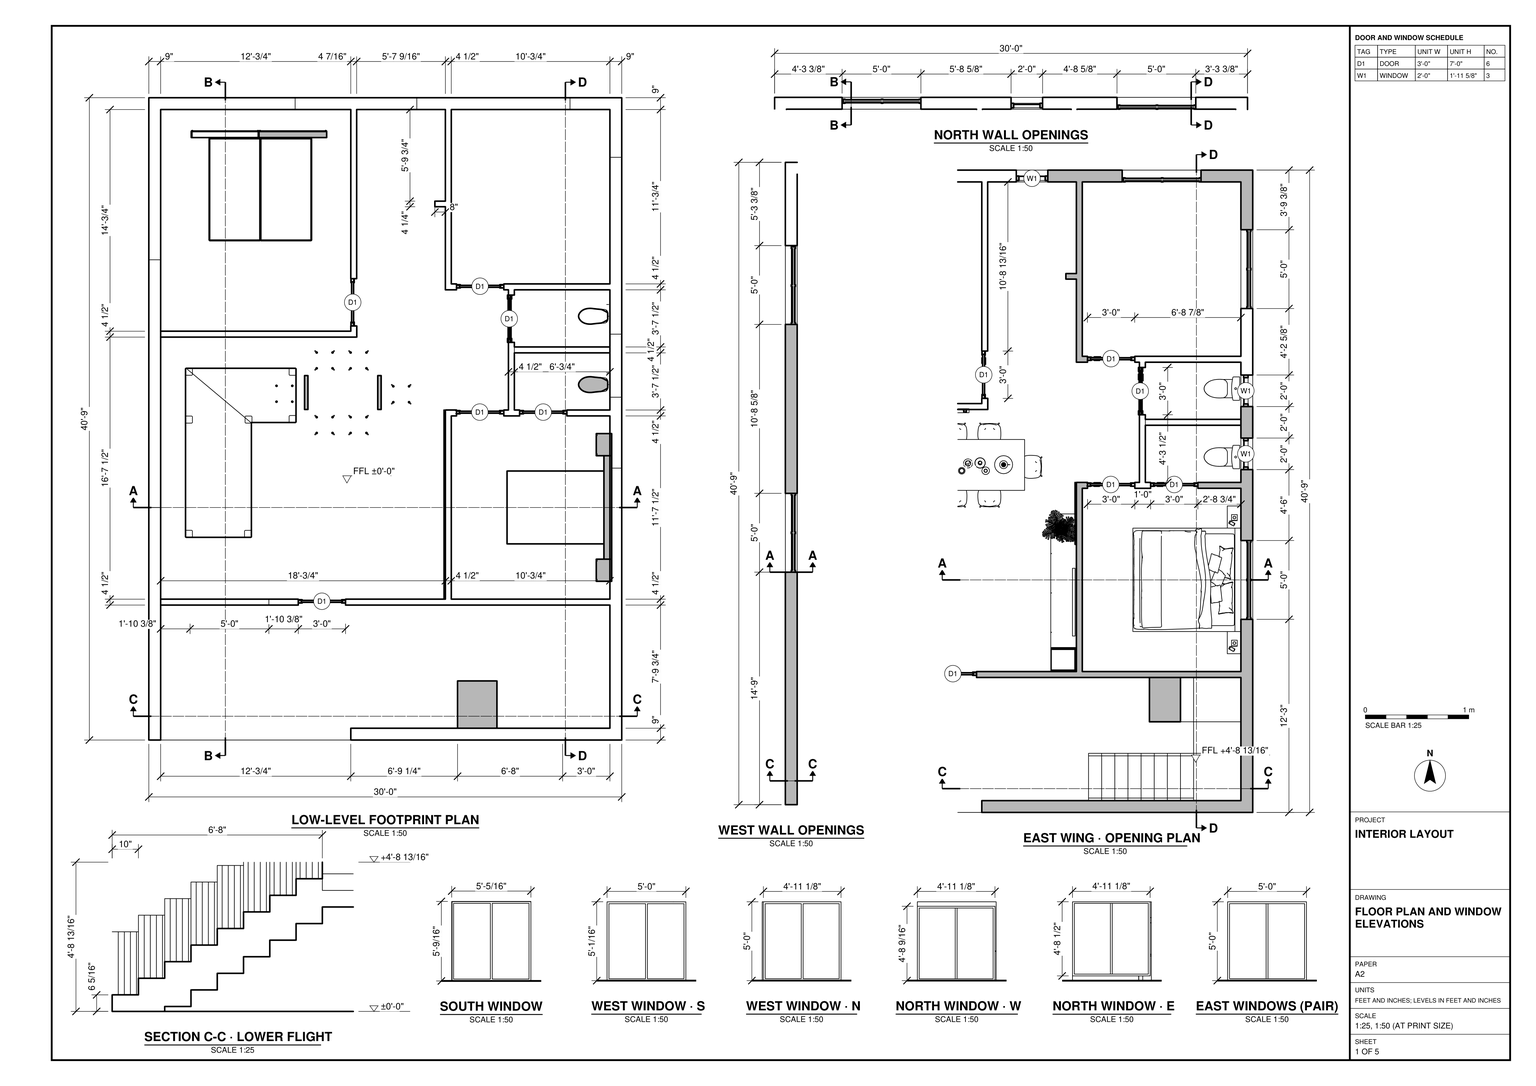
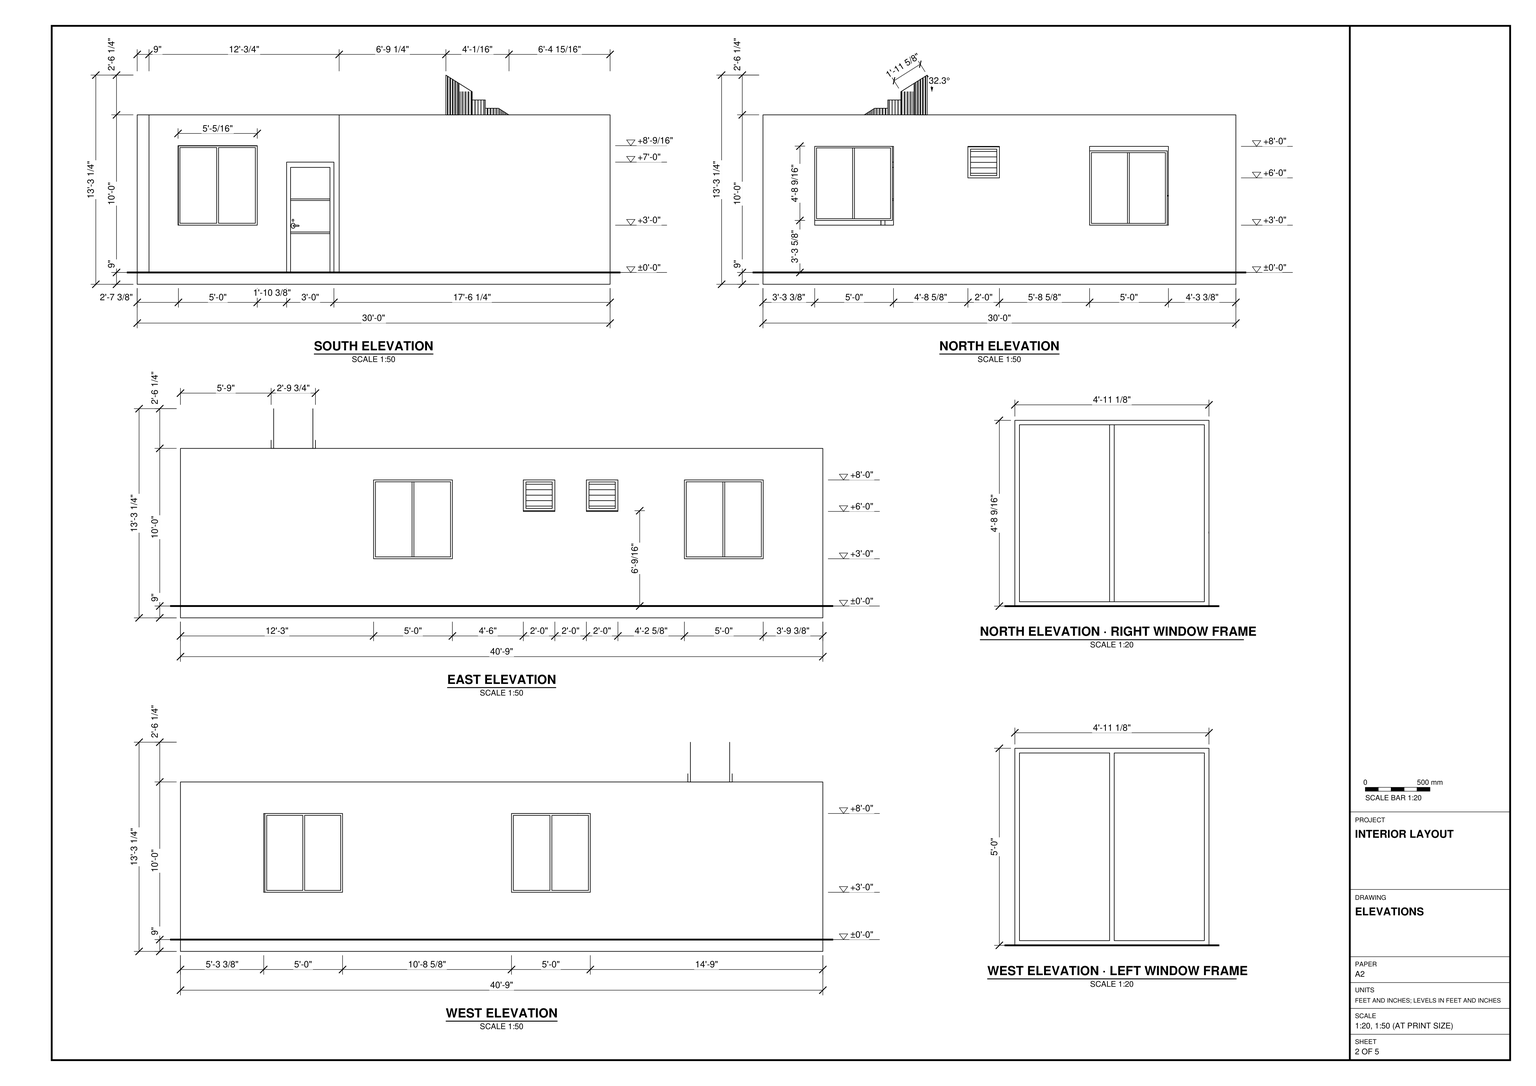
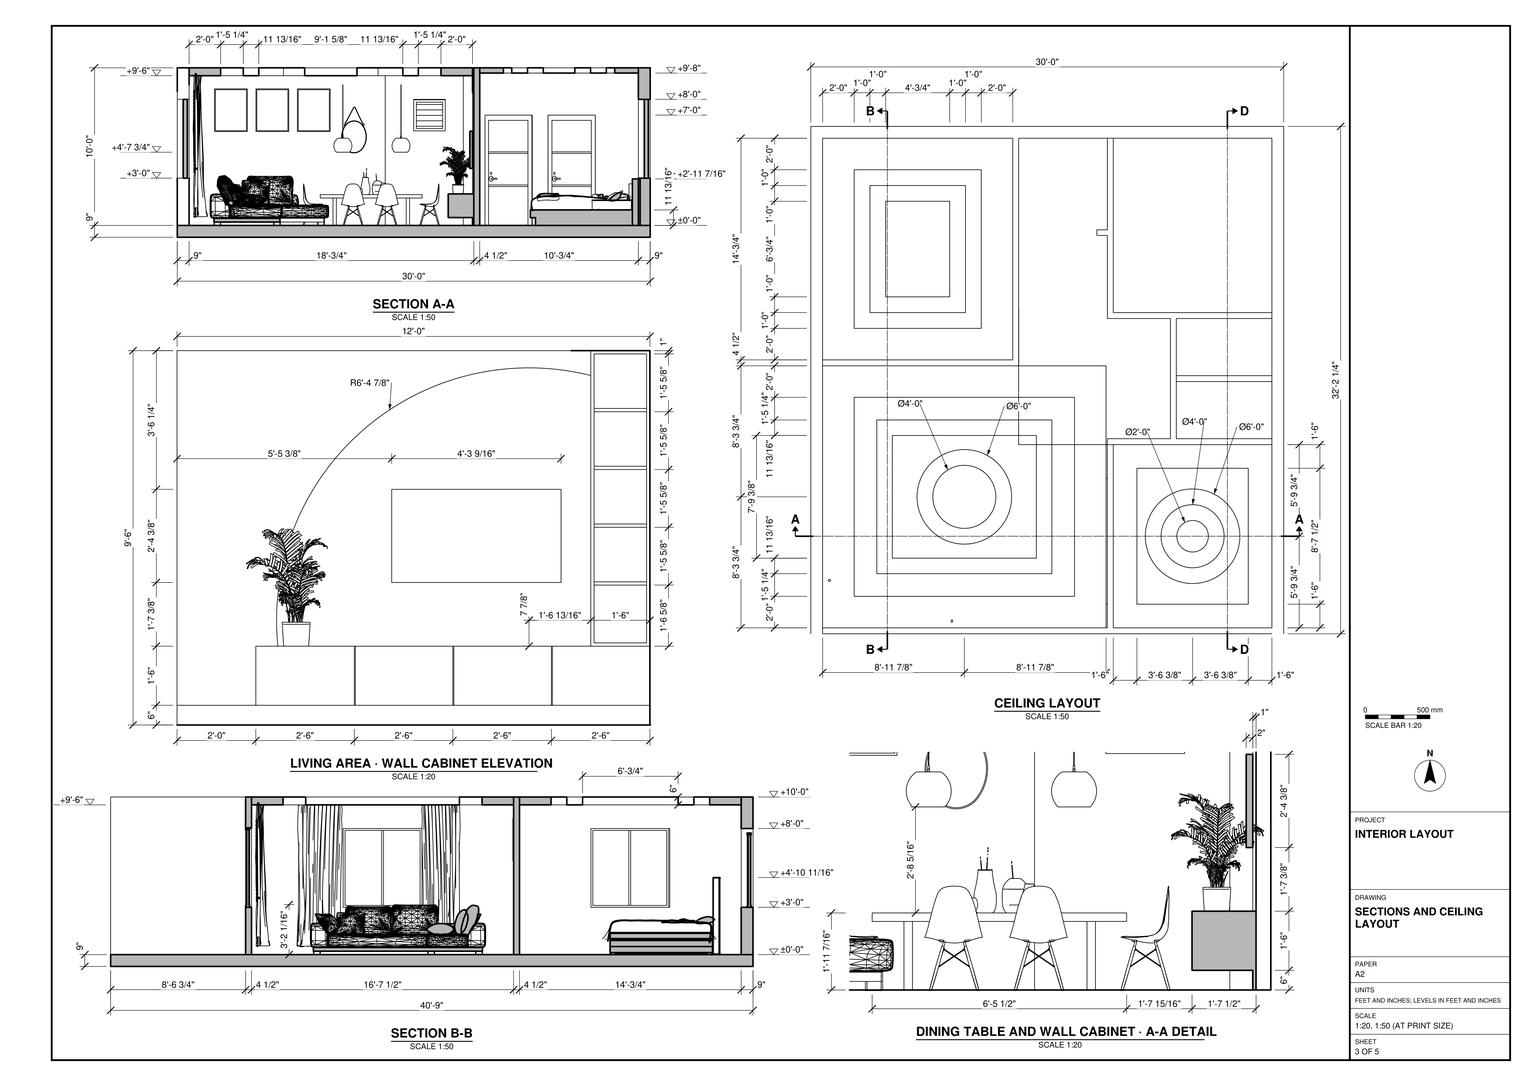
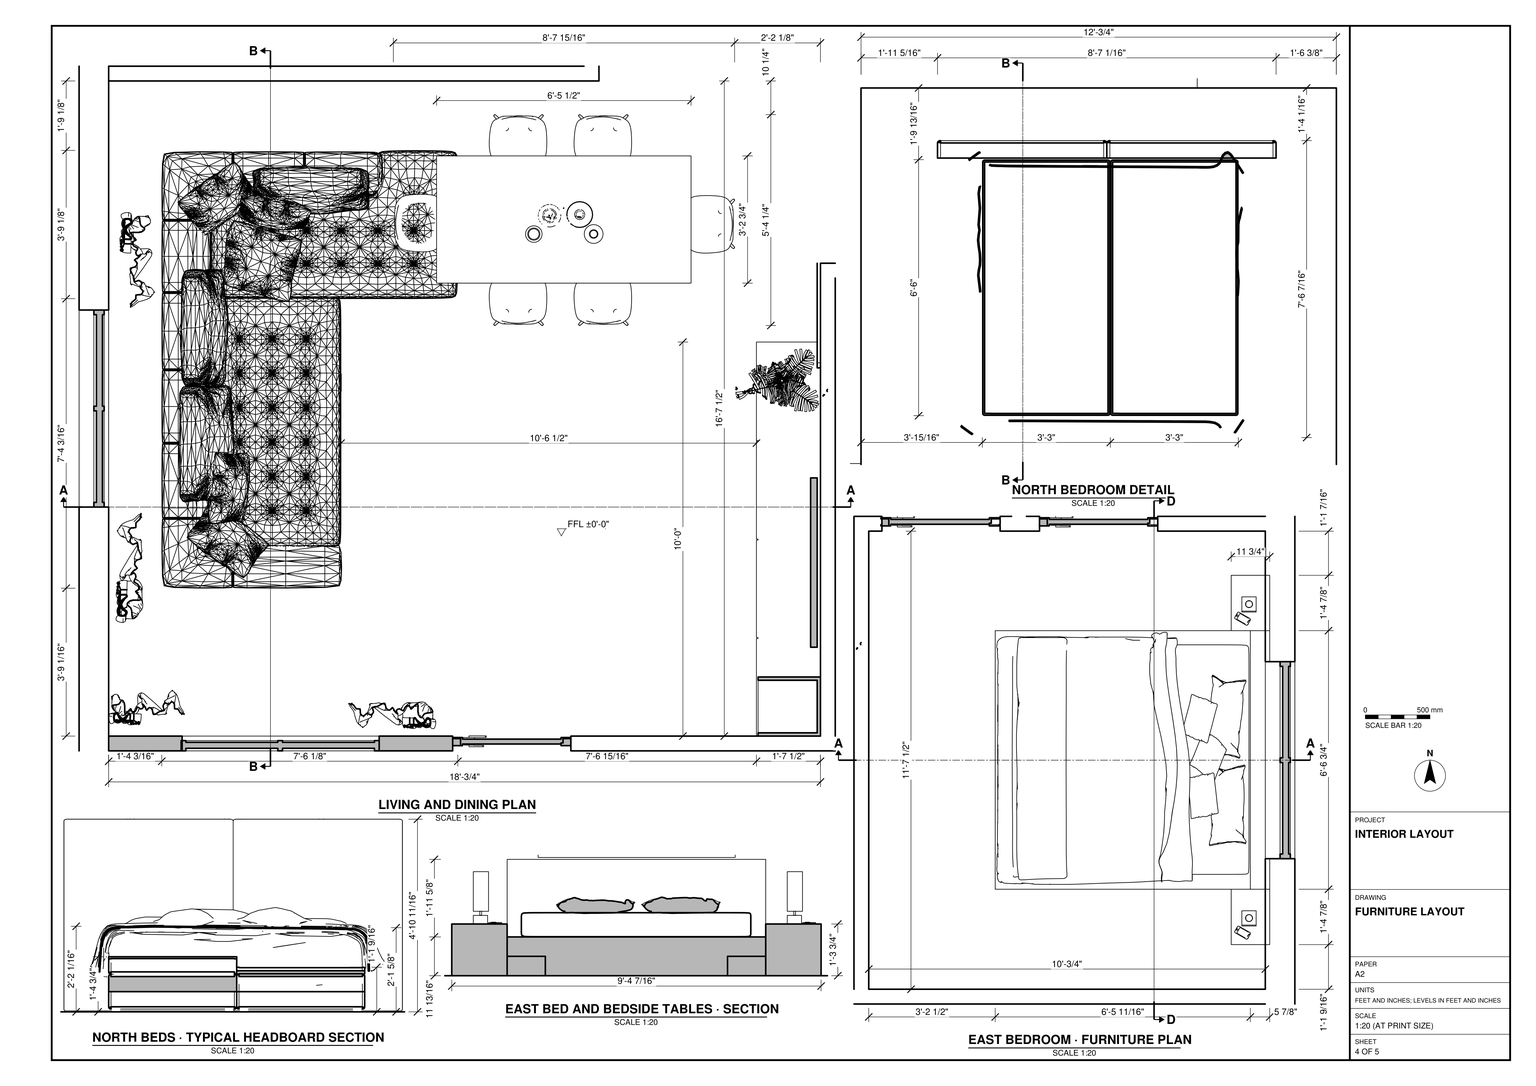
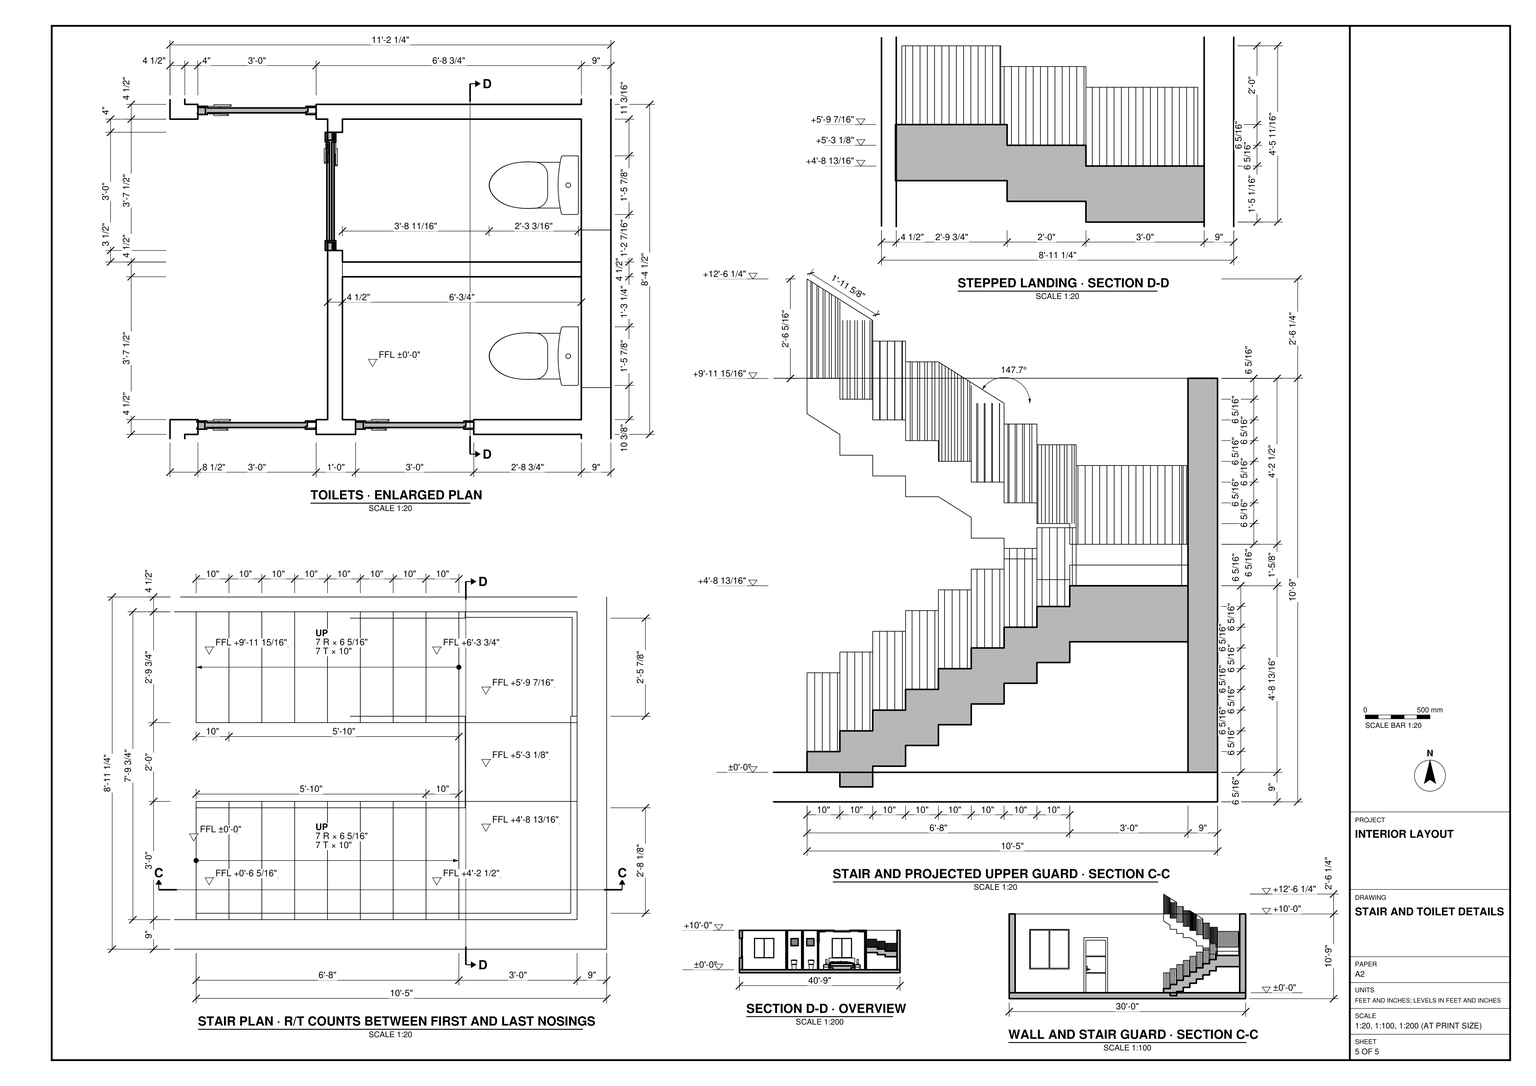
Build the single-storey interior in SketchUp from task_files/diagram_01.pdf. Work in feet and inches. Set the finished floor at ±0'-0" and make the overall model 30'-0" east to west, 40'-9" north to south and 10'-9" high.

Lay out the floor slab, perimeter walls and partitions using the thicknesses on the plan and sections. Keep the living and dining area open on the west side. Place the northwest bed against the north wall and the southeast bed against the east wall. Follow the east-wing plan for the northeast room, the two small toilet rooms and their doorways. Fit the doors and window units, using the elevations to distinguish the large two-panel windows from the smaller high-level openings. Model the lower stair flight, landing and railing in the southern entrance area.

Use the furniture footprints to place the L-shaped sofa, dining table and chairs. Build the living-area wall cabinet with its low cupboards, curved panel edge and tall shelving at one end. Model the flat roof and the changes in ceiling profile, including the nested rectangular and circular features shown in the ceiling plan. Decor and loose items may be any suitable library components.

Keep walls, slabs and roof in separate groups or components, do the same for each furniture or joinery piece, and use components for repeated parts. Save one SketchUp model as output_files/furnished_residential_interior_and_its_entrance_stair.skp.

# SketchUp Ruby script. Lengths in inches.
U = 1.inch
M = Sketchup.active_model
def pt(a) = Geom::Point3d.new(a.map { |v| v * U })
def face(e, loops, mat)
  f = e.add_face(loops[0].map { |a| pt(a) })
  loops[1..].each { |l| e.add_face(l.map { |a| pt(a) }).erase! }
  f.material = f.back_material = mat if mat
  f
end
# faces: each face lists its corners as indices into pts; further lists are holes
def faces(e, pts, list, mat = nil) = list.each { |f| face(e, (f[0].is_a?(Array) ? f : [f]).map { |l| l.map { |i| pts[i] } }, mat) }
# xy, xz, yz: faces in a plane at the given z, y or x. An outline is a flat list of corners, or four numbers for a rectangle; further outlines are holes
def ring(l) = l.size == 4 ? [[l[0], l[1]], [l[2], l[1]], [l[2], l[3]], [l[0], l[3]]] : l.each_slice(2).to_a
def flat(e, list, mat, &to3) = list.each { |f| face(e, (f[0].is_a?(Array) ? f : [f]).map { |l| ring(l).map { |u, v| to3.(u, v) } }, mat) }
def xy(e, z, list, mat = nil) = flat(e, list, mat) { |x, y| [x, y, z] }
def xz(e, y, list, mat = nil) = flat(e, list, mat) { |x, z| [x, y, z] }
def yz(e, x, list, mat = nil) = flat(e, list, mat) { |y, z| [x, y, z] }
def lines(e, pts, list) = list.each { |a, b| e.add_line(pt(pts[a]), pt(pts[b])) }
# prism: a flat outline (further loops are holes) pulled along v
def prism(e, loops, v, mat = nil)
  f = face(e, loops, mat); d = Geom::Vector3d.new(v.map { |x| x * U })
  f.pushpull(f.normal.samedirection?(d) ? d.length : -d.length)
end
def box(e, o, s, mat = nil) = prism(e, [[o, [o[0] + s[0], o[1], o[2]], [o[0] + s[0], o[1] + s[1], o[2]], [o[0], o[1] + s[1], o[2]]]], [0, 0, s[2]], mat)
def at(x, y, z, deg = 0) = Geom::Transformation.translation(pt([x, y, z])) * Geom::Transformation.rotation(ORIGIN, Z_AXIS, deg.degrees)
def axes(o, x, y, z) = Geom::Transformation.new([*x, 0, *y, 0, *z, 0, *pt(o).to_a, 1])
def part(name) = M.definitions.add(name)
# library, detail: a bought-in or finely detailed component or shape, given as its bounding box
def library(name, o, s) = part(name).tap { |d| box(d.entities, o, s) }
def detail(e, o, s) = box(e.add_group.entities, o, s)
def put(e, d, t, mat = nil) = e.add_instance(d, t).tap { |i| i.material = mat if mat }
def group(e, t, mat = nil) = e.add_group.tap { |g| g.transformation = t; g.material = mat if mat }.entities
root = M.entities
M.materials.add("F10").color = [176, 183, 172]
M.materials.add("F11").color = [173, 179, 169]
M.materials.add("F20").color = [169, 167, 158]
M.materials.add("Querkus Oak Naturel Adagio _ Architonic1").color = [173, 130, 81]
M.materials.add("[0010_Snow]").color = [255, 250, 250]
M.materials.add("[0035_Tan]").color = [210, 180, 140]
M.materials.add("[0057_DarkKhaki]").color = [189, 183, 107]
M.materials.add("[0072_DarkSeaGreen]").color = [143, 188, 143]
M.materials.add("[0110_LightSlateGray]").color = [119, 136, 153]
M.materials.add("[Carrera Marble]").color = [207, 207, 207]
M.materials.add("[Color_008]").color = [30, 30, 30]
M.materials.add("[Color_009]").color = [0, 0, 0]
M.materials.add("[Stone Vein Gray]").color = [166, 165, 165]
M.materials.add("[Translucent Glass Gray]").color = [128, 128, 128]
M.materials.add("[Translucent Glass Tinted]1").color = [7, 201, 240]
M.materials.add("[Translucent_Glass_Gray]").color = [128, 128, 128]
M.materials.add("[Wood Cherry Original]").color = [152, 86, 42]
M.materials.add("[Wood Floor Parquet]").color = [145, 89, 39]
c1 = library("main+door",[0,-0.79,0],[47.24,7.88,82.68])
c2 = library("Modern+dining",[-0.9,-1.38,-0.1],[126.72,78.33,130.86])
c3 = library("Senza",[-40.91,-66.2,-0.5],[133.3,90.15,38.26])
c4 = library("Bed",[-100.55,9.74,0],[90.43,103.1,58.68])
c5 = library("Platform bed",[0,0,0],[83.59,112.46,35.43])
c6 = library("CS300DRT",[0,0,0],[27.18,17.85,30.31])
c7 = library("SKT_Nearly Natural 5' Kentia Palm Silk Tree",[-23.18,-17.61,0],[47.48,43.95,59.125])
c8 = library("Curtains and rod",[2.63,-1.46,0.02],[153.32,14.02,114.15])
c9 = part("Group\#37")
prism(c9.entities,[[[0,0.6,0],[0,0.6,24.5],[19,0.6,24.5],[19,0.6,0]],[[0.5,0.6,0.5],[18.5,0.6,0.5],[18.5,0.6,24],[0.5,0.6,24]]],[0,-0.6,0])
c10 = part("F9")
g1 = group(c10.entities,at(48,0,0))
xy(g1,0.5,[[0.5,0.3,18.5,0.6]])
xy(g1,24,[[0.5,0.3,18.5,0.6]])
xz(g1,0.3,[[0.5,0.5,18.5,24]],"F11")
xz(g1,0.6,[[0.5,0.5,18.5,24]],"[0010_Snow]")
yz(g1,0.5,[[0.3,0.5,0.6,24]])
yz(g1,18.5,[[0.3,0.5,0.6,24]])
put(g1,c9,axes([19,0,0],[-1,0,0],[0,1,0],[0,0,1]),"Querkus Oak Naturel Adagio _ Architonic1")
g2 = group(c10.entities,at(24,0,0))
xy(g2,0.5,[[0.5,0.3,18.5,0.6]])
xy(g2,24,[[0.5,0.3,18.5,0.6]])
xz(g2,0.3,[[0.5,0.5,18.5,24]],"F10")
xz(g2,0.6,[[0.5,0.5,18.5,24]],"[0010_Snow]")
yz(g2,0.5,[[0.3,0.5,0.6,24]])
yz(g2,18.5,[[0.3,0.5,0.6,24]])
put(g2,c9,axes([19,0,0],[-1,0,0],[0,1,0],[0,0,1]),"Querkus Oak Naturel Adagio _ Architonic1")
g3 = group(c10.entities,at(0,0,0))
xy(g3,0.5,[[0.5,0.3,18.5,0.6]])
xy(g3,24,[[0.5,0.3,18.5,0.6]])
xz(g3,0.3,[[0.5,0.5,18.5,24]],"F20")
xz(g3,0.6,[[0.5,0.5,18.5,24]],"[0010_Snow]")
yz(g3,0.5,[[0.3,0.5,0.6,24]])
yz(g3,18.5,[[0.3,0.5,0.6,24]])
put(g3,c9,axes([19,0,0],[-1,0,0],[0,1,0],[0,0,1]),"Querkus Oak Naturel Adagio _ Architonic1")
c11 = library("Round wall hanging",[0,0,0],[26.88,1.18,49.49])
c12 = library("Group\#5",[0,0,0],[116.44,93.99,154.6875])
c13 = part("ventilator")
g4 = group(c13.entities,at(0,0,0))
xy(g4,0,[[0,0,24,1],[0,1,24,6.83]],"[Wood Floor Parquet]")
xy(g4,1.75,[[2,0,22,6.83]],"[Wood Floor Parquet]")
xy(g4,21.87,[[2,0,22,6.83]],"[Wood Cherry Original]")
xy(g4,23.62,[[0,0,24,1],[0,1,24,6.83]],"[Wood Floor Parquet]")
xz(g4,0,[[[0,0,24,23.62],[2,1.75,22,21.87]]],"[Wood Floor Parquet]")
xz(g4,6.83,[[[0,0,24,23.62],[2,1.75,22,21.87]]],"[Wood Cherry Original]")
yz(g4,0,[[0,0,1,23.62],[1,0,6.83,23.62]],"[Wood Floor Parquet]")
yz(g4,2,[[0,1.75,6.83,1.75,6.83,7.66,0,3.5],[0,3.5,6.83,7.66,6.83,11.8125,0,7.66],[0,7.66,6.83,11.8125,6.83,15.97,0,11.8125],[0,11.8125,6.83,15.97,6.83,20.12,0,15.97],[0,15.97,6.83,20.12,6.83,21.87,0,21.87]],"[Wood Floor Parquet]")
yz(g4,22,[[0,1.75,0,3.5,6.83,7.66,6.83,1.75],[0,3.5,0,7.66,6.83,11.8125,6.83,7.66],[0,7.66,0,11.8125,6.83,15.97,6.83,11.8125],[0,11.8125,0,15.97,6.83,20.12,6.83,15.97],[0,15.97,0,21.87,6.83,21.87,6.83,20.12]],"[Wood Floor Parquet]")
yz(g4,24,[[0,0,1,23.62],[1,0,6.83,23.62]],"[Wood Floor Parquet]")
p = [[2,0,3.5],[2,6.83,7.66],[22,6.83,7.66],[22,0,3.5],[2,6.83,11.8125],[2,0,7.66],
  [22,0,7.66],[22,6.83,11.8125],[2,0,11.8125],[2,6.83,15.97],[22,6.83,15.97],[22,0,11.8125],
  [2,6.83,20.12],[2,0,15.97],[22,0,15.97],[22,6.83,20.12]]
faces(g4,p,[[0,1,2,3],[4,5,6,7],[8,9,10,11]],"[Translucent Glass Tinted]1")
faces(g4,p,[[12,13,14,15]],"[Translucent Glass Gray]")
c14 = part("Group\#2")
xy(c14.entities,0,[[0,0,82.68,1.18]],"[Color_009]")
xy(c14.entities,1.97,[[1.97,0.98,40.35,1.18],[42.32,0.98,80.71,1.18]])
xy(c14.entities,1.97,[[1.97,0,40.35,0.3],[42.32,0,80.71,0.3]],"[Color_009]")
xy(c14.entities,80.71,[[1.97,0,40.35,0.3],[42.32,0,80.71,0.3],[1.97,0.3,40.35,0.98],[42.32,0.3,80.71,0.98],[1.97,0.98,40.35,1.18],
  [42.32,0.98,80.71,1.18]])
xy(c14.entities,82.68,[[0,0,82.68,1.18]],"[Color_008]")
xz(c14.entities,0,[[[0,0,82.68,82.68],[1.97,1.97,40.35,80.71],[42.32,1.97,80.71,80.71]]],"[Color_009]")
xz(c14.entities,0.3,[[1.97,1.97,40.35,80.71],[42.32,1.97,80.71,80.71]],"[Translucent_Glass_Gray]")
xz(c14.entities,0.98,[[1.97,1.97,40.35,80.71],[42.32,1.97,80.71,80.71]],"[Translucent_Glass_Gray]")
xz(c14.entities,1.18,[[[0,0,82.68,82.68],[1.97,1.97,80.71,80.71]],[40.35,1.97,42.32,80.71]],"[Color_009]")
yz(c14.entities,0,[[0,0,1.18,82.68]],"[Color_009]")
yz(c14.entities,1.97,[[0.98,1.97,1.18,80.71]])
yz(c14.entities,1.97,[[0,1.97,0.3,80.71]],"[Color_009]")
yz(c14.entities,40.35,[[0,1.97,0.3,80.71],[0.98,1.97,1.18,80.71]],"[Color_009]")
yz(c14.entities,42.32,[[0,1.97,0.3,80.71],[0.98,1.97,1.18,80.71]])
yz(c14.entities,80.71,[[0,1.97,0.3,80.71],[0.98,1.97,1.18,80.71]],"[Color_009]")
yz(c14.entities,82.68,[[0,0,1.18,82.68]],"[Color_009]")
c15 = library("Group\#28",[0,0,0],[19.5,144,120])
c16 = library("Group\#36",[0,0,-6],[215.75,199.5,6])
c17 = library("Group\#42",[0,0,-4],[120.75,139.5,4])
xy(root,120,[[158.21,246.75,351,246.75,351,347.25,230.25,347.25,230.25,480,158.21,480],[230.25,347.25,351,480]])
# 2 loose lines left out
put(root,c1,axes([282.21,248.34,0],[0.762,0,0],[0,0.42,0],[0,0,1.016]))
put(root,c1,axes([233.96,248.34,0],[0.762,0,0],[0,0.42,0],[0,0,1.016]))
put(root,c1,axes([273.75,338.75,0],[0,-0.762,0],[0.42,0,0],[0,0,1.016]))
put(root,c2,axes([96.43,233.41,-0.1],[0.82,0,0],[0,0.82,0],[0,0,0.82]))
put(root,c3,at(49.13,193.21,0.31,90))
put(root,c4,at(22.55,363.42,0,-90))
put(root,c5,at(268.76,120.84,0))
put(root,c6,at(350.09,331.57,0,180))
put(root,c6,at(350.09,279.51,0,180))
put(root,c7,axes([213.79,214.89,23.75],[0.65,0,0],[0,0.65,0],[0,0,0.65]))
put(root,c8,axes([7.29,108.71,5.83],[0.65,0,0],[0,1,0],[0,0,1]))
put(root,c8,axes([10.46,268.91,5.83],[0,-0.8151,0],[1,0,0],[0,0,1]))
put(root,c10,axes([28.35,306.15,71.47],[1.3144,0,0],[0,1.24,0],[0,0,1.3268]))
put(root,c11,axes([124.94,304.29,55.15],[0.71,0,0],[0,2.5702,0],[0,0,0.71]))
put(root,c12,at(235,9,-4.4375))
g5 = group(root,at(0,0,-9))
xy(g5,0,[[0,0,360,489]])
xy(g5,9,[[0,0,360,489]],"[Stone Vein Gray]")
xz(g5,0,[[0,0,360,9]])
xz(g5,489,[[0,0,360,9]])
yz(g5,0,[[0,0,489,9]])
yz(g5,360,[[0,0,489,9]])
g6 = group(root,at(0,0,0))
xy(g6,0,[[0,0,9,177],[153.75,0,153.75,9,351,9,351,102.75,149.75,102.75,149.75,107.25,225.75,107.25,225.75,251.25,234.25,251.25,234.25,246.75,230.25,246.75,230.25,107.25,351,107.25,351,207,360,207,360,0],[9,102.75,91.375,107.25],[91.375,102.75,113.75,107.25],[0,177,9,365.625],
  [351,207,351,246.75,318.25,246.75,318.25,251.25,351,251.25,351,261,360,261,360,207],[270.25,246.75,270.25,251.25,273.75,251.25,273.75,302.75,278.25,302.75,278.25,251.25,282.25,251.25,282.25,246.75],[351,261,360,309],[9,306.75,9,311.25,153.75,311.25,153.75,315.25,158.3,315.25,158.3,306.75],[351,309,351,342.75,278.25,342.75,278.25,338.75,273.75,338.75,273.75,342.75,270.25,342.75,270.25,347.25,351,347.25,351,443.625,360,443.625,360,309],
  [225.75,342.75,225.75,406.01,217.75,406.01,217.75,410.25,225.75,410.25,225.75,480,204,480,204,489,320.625,489,320.625,480,230.25,480,230.25,347.25,234.23,347.25,234.23,342.75],[153.75,351.25,153.75,480,111.375,480,111.375,489,204,489,204,480,158.21,480,158.21,351.25],[0,365.625,0,489,111.375,489,111.375,480,9,480,9,365.625],[351,443.625,351,480,320.625,480,320.625,489,360,489,360,443.625]])
xy(g6,36,[[31.375,102.75,91.375,107.25],[351,147,360,207],[0,177,9,237],[0,365.625,9,425.625],[351,383.625,360,443.625],
  [51.375,480,111.375,489],[260.625,480,320.625,489]])
xy(g6,72,[[351,261,360,285],[351,309,360,333],[180,480,204,489]])
xy(g6,84,[[113.75,102.75,149.75,107.25],[234.25,246.75,270.25,251.25],[282.25,246.75,318.25,251.25],[273.75,302.75,278.25,338.75],[153.75,315.25,158.21,351.25],
  [158.21,315.25,158.3,351.25],[234.23,342.75,270.25,347.25]])
xy(g6,96,[[351,147,360,207],[0,177,9,237],[351,261,360,285],[351,309,360,333],[0,365.625,9,425.625],
  [351,383.625,360,443.625],[51.375,480,111.375,489],[180,480,204,489],[260.625,480,320.625,489]])
xy(g6,96.36,[[31.375,102.75,91.375,107.25]])
xy(g6,120,[[[0,0,9,0,9,480,153.75,480,153.75,311.25,9,311.25,9,306.75,158.3,306.75,158.3,351.25,158.21,351.25,158.21,480,225.75,480,225.75,410.25,217.75,410.25,217.75,406.01,225.75,406.01,225.75,342.75,273.75,342.75,273.75,251.25,225.75,251.25,225.75,107.25,9,107.25,9,102.75,351,102.75,351,9,153.75,9,153.75,0,360,0,360,489,0,489],[230.25,107.25,351,246.75],[230.25,347.25,351,480],[278.25,251.25,351,342.75]],[278.25,294.75,351,299.25]])
xz(g6,0,[[0,0,9,120],[153.75,0,360,120]])
xz(g6,9,[[153.75,0,351,120]])
xz(g6,102.75,[[[9,0,113.75,0,113.75,84,149.75,84,149.75,0,351,0,351,120,9,120],[31.375,36,91.375,96.36]]])
xz(g6,107.25,[[91.375,0,91.375,120,225.75,120,225.75,0,149.75,0,149.75,84,113.75,84,113.75,0],[230.25,0,351,120]],"[0035_Tan]")
xz(g6,107.25,[[9,0,9,120,91.375,120,91.375,96.36,31.375,96.36,31.375,36,91.375,36,91.375,0]],"[0057_DarkKhaki]")
xz(g6,147,[[351,36,360,96]])
xz(g6,177,[[0,36,9,96]])
xz(g6,207,[[351,36,360,96]])
xz(g6,237,[[0,36,9,96]])
xz(g6,246.75,[[230.25,0,234.25,0,234.25,84,270.25,84,270.25,0,282.25,0,282.25,84,318.25,84,318.25,0,351,0,351,120,230.25,120]],"[0035_Tan]")
xz(g6,251.25,[[270.25,0,273.75,120]])
xz(g6,251.25,[[225.75,0,225.75,120,270.25,120,270.25,84,234.25,84,234.25,0],[278.25,0,278.25,120,318.25,120,318.25,84,282.25,84,282.25,0],[318.25,0,351,120]],"[0035_Tan]")
xz(g6,261,[[351,72,360,96]])
xz(g6,285,[[351,72,360,96]])
xz(g6,294.75,[[278.25,0,351,120]],"[0035_Tan]")
xz(g6,299.25,[[278.25,0,351,120]],"[0035_Tan]")
xz(g6,302.75,[[273.75,0,278.25,84]])
xz(g6,306.75,[[9,0,158.3,120]],"[0035_Tan]")
xz(g6,309,[[351,72,360,96]])
xz(g6,311.25,[[9,0,153.75,120]],"[0035_Tan]")
xz(g6,315.25,[[153.75,0,158.3,84]])
xz(g6,333,[[351,72,360,96]])
xz(g6,338.75,[[273.75,0,278.25,84]])
xz(g6,342.75,[[225.75,0,234.23,0,234.23,84,270.25,84,270.25,0,273.75,0,273.75,120,225.75,120],[278.25,0,351,120]],"[0035_Tan]")
xz(g6,347.25,[[230.25,0,230.25,120,351,120,351,0,270.25,0,270.25,84,234.23,84,234.23,0]],"[0035_Tan]")
xz(g6,351.25,[[153.75,0,158.21,84],[158.21,84,158.3,120]])
xz(g6,365.625,[[0,36,9,96]])
xz(g6,383.625,[[351,36,360,96]])
xz(g6,406.01,[[217.75,0,225.75,120]])
xz(g6,410.25,[[217.75,0,225.75,120]])
xz(g6,425.625,[[0,36,9,96]])
xz(g6,443.625,[[351,36,360,96]])
xz(g6,480,[[[9,0,153.75,120],[51.375,36,111.375,96]],[[158.21,0,225.75,120],[180,72,204,96]],[[230.25,0,351,120],[260.625,36,320.625,96]]],"[0035_Tan]")
xz(g6,489,[[[0,0,360,120],[260.625,36,320.625,96],[51.375,36,111.375,96],[180,72,204,96]]])
yz(g6,0,[[[0,0,489,120],[365.625,36,425.625,96],[177,36,237,96]]])
yz(g6,9,[[0,0,102.75,120],[102.75,0,107.25,120],[306.75,0,311.25,120]])
yz(g6,9,[[[107.25,0,306.75,120],[177,36,237,96]],[[311.25,0,480,120],[365.625,36,425.625,96]]],"[0035_Tan]")
yz(g6,31.375,[[102.75,36,107.25,96.36]])
yz(g6,51.375,[[480,36,489,96]])
yz(g6,91.375,[[102.75,36,107.25,96.36]])
yz(g6,111.375,[[480,36,489,96]])
yz(g6,113.75,[[102.75,0,107.25,84]])
yz(g6,149.75,[[102.75,0,107.25,84]])
yz(g6,153.75,[[0,0,9,120]])
yz(g6,153.75,[[311.25,0,311.25,120,480,120,480,0,351.25,0,351.25,84,315.25,84,315.25,0]],"[0035_Tan]")
yz(g6,158.21,[[351.25,0,480,120]],"[0035_Tan]")
yz(g6,158.3,[[306.75,0,315.25,0,315.25,84,351.25,84,351.25,120,306.75,120]],"[0035_Tan]")
yz(g6,180,[[480,72,489,96]])
yz(g6,204,[[480,72,489,96]])
yz(g6,217.75,[[406.01,0,410.25,120]])
yz(g6,225.75,[[342.75,0,406.01,120],[410.25,0,480,120]],"[0035_Tan]")
yz(g6,225.75,[[107.25,0,251.25,120]],"[Carrera Marble]")
yz(g6,230.25,[[347.25,0,480,120]],"[0035_Tan]")
yz(g6,230.25,[[107.25,0,246.75,120]],"[0072_DarkSeaGreen]")
yz(g6,234.23,[[342.75,0,347.25,84]])
yz(g6,234.25,[[246.75,0,251.25,84]])
yz(g6,260.625,[[480,36,489,96]])
yz(g6,270.25,[[246.75,0,251.25,84],[342.75,0,347.25,84]])
yz(g6,273.75,[[251.25,0,251.25,120,342.75,120,342.75,0,338.75,0,338.75,84,302.75,84,302.75,0]],"[0035_Tan]")
yz(g6,278.25,[[251.25,0,294.75,120],[299.25,0,302.75,0,302.75,84,338.75,84,338.75,0,342.75,0,342.75,120,299.25,120]],"[0072_DarkSeaGreen]")
yz(g6,282.25,[[246.75,0,251.25,84]])
yz(g6,318.25,[[246.75,0,251.25,84]])
yz(g6,320.625,[[480,36,489,96]])
yz(g6,351,[[9,0,102.75,120],[294.75,0,299.25,120]])
yz(g6,351,[[[107.25,0,246.75,120],[147,36,207,96]],[[251.25,0,294.75,120],[261,72,285,96]],[[299.25,0,342.75,120],[309,72,333,96]],[[347.25,0,480,120],[383.625,36,443.625,96]]],"[0035_Tan]")
yz(g6,360,[[[0,0,489,120],[383.625,36,443.625,96],[147,36,207,96],[261,72,285,96],[309,72,333,96]]])
put(g6,c13,axes([356.45,261,72.58],[0,1,0],[-0.5,0,0],[0,0,1]))
put(g6,c1,axes([273.02,338.75,0],[0,-0.762,0],[0.42,0,0],[0,0,1.016]))
put(g6,c1,axes([153.875,351.21,0],[0,-0.762,0],[0.42,0,0],[0,0,1.016]))
put(g6,c1,axes([113.75,104.34,0],[0.762,0,0],[0,0.42,0],[0,0,1.016]))
put(g6,c13,axes([356.45,309,72.58],[0,1,0],[-0.5,0,0],[0,0,1]))
put(g6,c13,axes([204,484.5,72],[-1,0,0],[0,-0.5,0],[0,0,1]))
put(g6,c1,axes([234.14,344.17,0],[0.762,0,0],[0,0.42,0],[0,0,1.016]))
put(g6,c14,axes([52.26,484.5,36],[0.715,0,0],[0,2.65,0],[0,0,0.6844]))
put(g6,c14,axes([4.5,237,36],[0,-0.72571,0],[2.65,0,0],[0,0,0.72546]))
put(g6,c14,axes([31.08,102.75,36],[0.7293,0,0],[0,2.65,0],[0,0,0.73231]))
put(g6,c14,axes([355.5,207,36],[0,-0.72571,0],[2.65,0,0],[0,0,0.72571]))
put(g6,c14,axes([355.5,443.625,36],[0,-0.72571,0],[2.65,0,0],[0,0,0.72571]))
put(g6,c14,axes([4.5,424.74,36],[0,-0.715,0],[2.65,0,0],[0,0,0.72571]))
put(g6,c14,axes([261.51,480,39.6],[0.715,0,0],[0,2.65,0],[0,0,0.6844]))
put(root,c15,at(206.25,107.25,0))
put(root,c16,at(9,107.25,120))
g7 = group(root,at(9,311.25,120))
xy(g7,-6,[[[0,0,144.75,168.75],[24,24,120.75,144.75]],[[36,36,108.75,132.75],[48,48,96.75,120.75]]],"[0110_LightSlateGray]")
xy(g7,0,[[[0,0,144.75,168.75],[24,24,120.75,144.75]],[[24,24,120.75,144.75],[36,36,108.75,132.75]],[48,48,96.75,120.75]])
xz(g7,0,[[0,-6,144.75,0]])
xz(g7,24,[[24,-6,120.75,0]])
xz(g7,36,[[36,-6,108.75,0]])
xz(g7,48,[[48,-6,96.75,0]])
xz(g7,120.75,[[48,-6,96.75,0]])
xz(g7,132.75,[[36,-6,108.75,0]])
xz(g7,144.75,[[24,-6,120.75,0]])
xz(g7,168.75,[[0,-6,144.75,0]])
yz(g7,0,[[0,-6,168.75,0]])
yz(g7,24,[[24,-6,144.75,0]])
yz(g7,36,[[36,-6,132.75,0]])
yz(g7,48,[[48,-6,120.75,0]])
yz(g7,96.75,[[48,-6,120.75,0]])
yz(g7,108.75,[[36,-6,132.75,0]])
yz(g7,120.75,[[24,-6,144.75,0]])
yz(g7,144.75,[[0,-6,168.75,0]])
put(root,c17,at(230.25,107.25,120))
